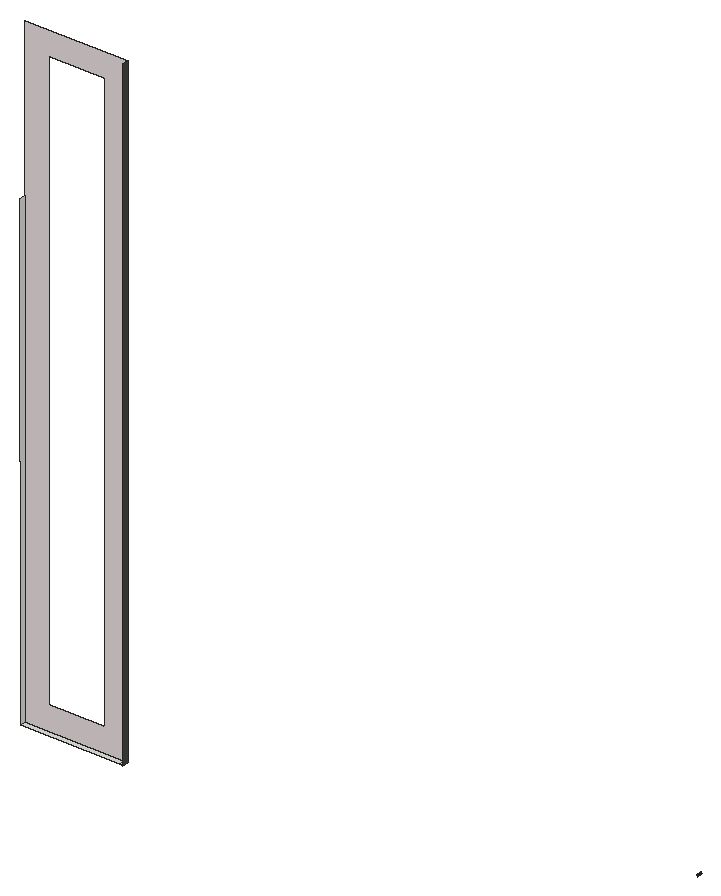
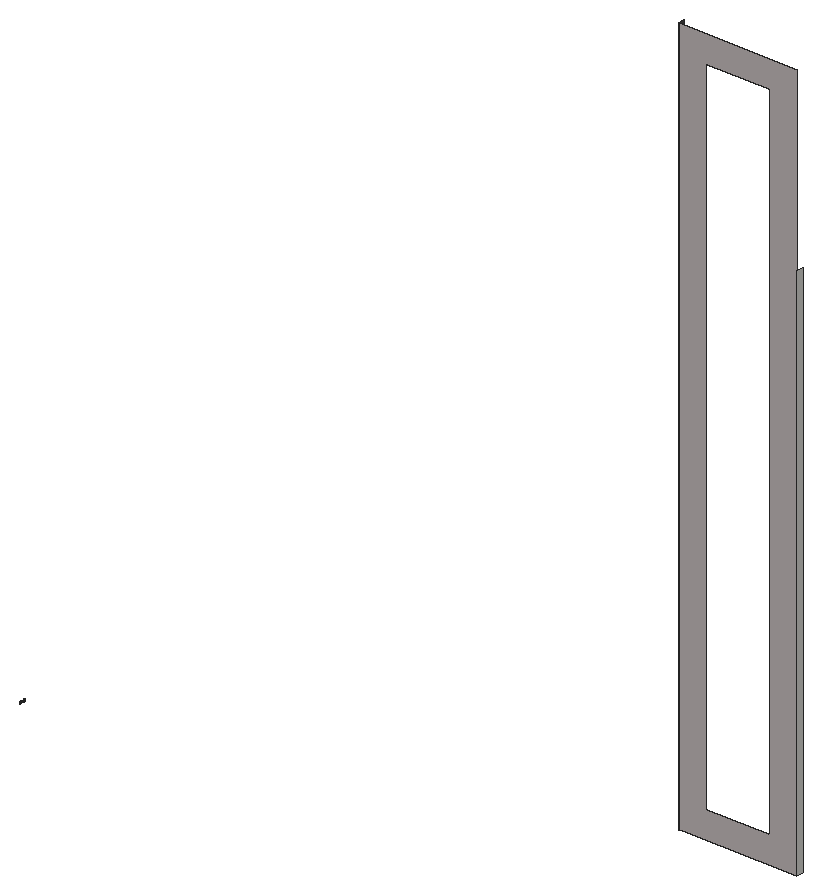
# SketchUp Ruby script. Lengths in inches.
U = 1.inch
M = Sketchup.active_model
def pt(a) = Geom::Point3d.new(a.map { |v| v * U })
def face(e, loops, mat)
  f = e.add_face(loops[0].map { |a| pt(a) })
  loops[1..].each { |l| e.add_face(l.map { |a| pt(a) }).erase! }
  f.material = f.back_material = mat if mat
  f
end
# faces: each face lists its corners as indices into pts; further lists are holes
def faces(e, pts, list, mat = nil) = list.each { |f| face(e, (f[0].is_a?(Array) ? f : [f]).map { |l| l.map { |i| pts[i] } }, mat) }
# xy, xz, yz: faces in a plane at the given z, y or x. An outline is a flat list of corners, or four numbers for a rectangle; further outlines are holes
def ring(l) = l.size == 4 ? [[l[0], l[1]], [l[2], l[1]], [l[2], l[3]], [l[0], l[3]]] : l.each_slice(2).to_a
def flat(e, list, mat, &to3) = list.each { |f| face(e, (f[0].is_a?(Array) ? f : [f]).map { |l| ring(l).map { |u, v| to3.(u, v) } }, mat) }
def xy(e, z, list, mat = nil) = flat(e, list, mat) { |x, y| [x, y, z] }
def xz(e, y, list, mat = nil) = flat(e, list, mat) { |x, z| [x, y, z] }
def yz(e, x, list, mat = nil) = flat(e, list, mat) { |y, z| [x, y, z] }
def lines(e, pts, list) = list.each { |a, b| e.add_line(pt(pts[a]), pt(pts[b])) }
# prism: a flat outline (further loops are holes) pulled along v
def prism(e, loops, v, mat = nil)
  f = face(e, loops, mat); d = Geom::Vector3d.new(v.map { |x| x * U })
  f.pushpull(f.normal.samedirection?(d) ? d.length : -d.length)
end
def box(e, o, s, mat = nil) = prism(e, [[o, [o[0] + s[0], o[1], o[2]], [o[0] + s[0], o[1] + s[1], o[2]], [o[0], o[1] + s[1], o[2]]]], [0, 0, s[2]], mat)
def at(x, y, z, deg = 0) = Geom::Transformation.translation(pt([x, y, z])) * Geom::Transformation.rotation(ORIGIN, Z_AXIS, deg.degrees)
def axes(o, x, y, z) = Geom::Transformation.new([*x, 0, *y, 0, *z, 0, *pt(o).to_a, 1])
def part(name) = M.definitions.add(name)
# library, detail: a bought-in or finely detailed component or shape, given as its bounding box
def library(name, o, s) = part(name).tap { |d| box(d.entities, o, s) }
def detail(e, o, s) = box(e.add_group.entities, o, s)
def put(e, d, t, mat = nil) = e.add_instance(d, t).tap { |i| i.material = mat if mat }
def group(e, t, mat = nil) = e.add_group.tap { |g| g.transformation = t; g.material = mat if mat }.entities
root = M.entities
M.materials.add("Generic\#1").color = [73, 71, 71]
M.materials.add("Generic\#5").color = [232, 222, 222]
M.materials.add("Material \#1").color = [140, 140, 140]
xy(root,30.535,[[34.973,39.25,88.165,42.5],[88.165,39.25,90.291,42.5]])
xy(root,30.853,[[337.189,118.4375,337.249,118.786,337.189,118.786]],"Material \#1")
xz(root,42.5,[[[34.973,30.535,90.291,30.535,90.279,368.38,34.912,368.38,34.917,283.879],[47.667,43.231,47.614,283.881,47.609,355.683,77.584,355.683,77.594,43.231]]],"Generic\#5")
xz(root,116.525,[[337.219,29.939,337.096,30,337.341,30],[337.219,29.939,337.15,29.955,337.096,30],[337.219,29.939,337.183,29.943,337.15,29.955],[337.15,29.955,337.121,29.974,337.096,30],[337.341,30,336.94,30.643,337.025,30.52],
  [337.341,30,337.056,30.439,336.94,30.643],[337.096,30,337.061,30.42,337.341,30],[337.096,30,337.062,30.414,337.061,30.42],[337.096,30,337.066,30.064,337.062,30.414],[337.096,30,337.078,30.03,337.066,30.064],
  [337.341,30,337.11,30.45,337.162,30.431],[337.066,30.064,337.062,30.102,337.062,30.414],[337.056,30.439,337.052,30.444,336.94,30.643],[337.052,30.444,337.048,30.45,336.94,30.643],[337.048,30.45,336.994,30.507,336.94,30.643],
  [337.048,30.45,337.043,30.455,336.994,30.507],[337.043,30.455,337.017,30.479,336.994,30.507],[336.994,30.507,336.959,30.57,336.94,30.643],[336.994,30.507,336.975,30.537,336.959,30.57],[337.025,30.52,336.94,30.643,336.996,30.568],
  [336.996,30.568,336.94,30.643,336.978,30.622],[336.959,30.57,336.948,30.606,336.94,30.643],[336.978,30.622,336.94,30.643,336.971,30.681],[336.94,30.643,336.938,30.681,336.945,30.748],[336.94,30.643,336.945,30.748,337,30.864],
  [336.94,30.643,336.978,30.74,336.971,30.681],[336.94,30.643,337,30.864,336.978,30.74],[336.978,30.74,337,30.864,336.996,30.795],[336.945,30.748,336.967,30.81,337,30.864],[336.996,30.795,337,30.864,337.025,30.842],
  [337.025,30.842,337,30.864,337.064,30.882],[337,30.864,337.043,30.909,337.095,30.944],[337,30.864,337.095,30.944,337.219,30.973],[337,30.864,337.11,30.913,337.064,30.882],[337,30.864,337.219,30.973,337.11,30.913],
  [337.11,30.913,337.219,30.973,337.162,30.932],[337.162,30.932,337.219,30.973,337.219,30.939],[337.095,30.944,337.154,30.966,337.219,30.973]],"Material \#1")
xz(root,116.862,[[337.207,30.51,337.195,30.535,337.231,30.535],[337.207,30.51,337.231,30.535,337.243,30.51],[337.195,30.535,337.189,30.544,337.237,30.544],[337.195,30.535,337.237,30.544,337.231,30.535],[337.189,30.544,337.189,30.563,337.237,30.563],
  [337.189,30.544,337.237,30.563,337.237,30.544],[337.189,30.563,337.195,30.572,337.231,30.572],[337.189,30.563,337.231,30.572,337.237,30.563],[337.195,30.572,337.195,30.604,337.243,30.604],[337.195,30.572,337.243,30.604,337.231,30.572],
  [337.195,30.604,337.195,30.634,337.243,30.634],[337.195,30.604,337.243,30.634,337.243,30.604],[337.195,30.634,337.186,30.658,337.252,30.658],[337.195,30.634,337.252,30.658,337.243,30.634],[337.186,30.658,337.186,30.683,337.252,30.683],
  [337.186,30.658,337.252,30.683,337.252,30.658],[337.186,30.683,337.195,30.707,337.243,30.707],[337.186,30.683,337.243,30.707,337.252,30.683],[337.195,30.707,337.189,30.724,337.249,30.724],[337.195,30.707,337.249,30.724,337.243,30.707],
  [337.189,30.724,337.189,30.78,337.249,30.78],[337.189,30.724,337.249,30.78,337.249,30.724],[337.189,30.78,337.196,30.784,337.241,30.784],[337.189,30.78,337.241,30.784,337.249,30.78],[337.196,30.784,337.196,30.793,337.241,30.793],
  [337.196,30.784,337.241,30.793,337.241,30.784],[337.196,30.793,337.189,30.797,337.249,30.797],[337.196,30.793,337.249,30.797,337.241,30.793],[337.189,30.797,337.189,30.853,337.249,30.853],[337.189,30.797,337.249,30.853,337.249,30.797]],"Material \#1")
xz(root,116.9,[[337.219,29.939,337.15,29.955,337.183,29.943],[337.15,29.955,337.062,30.414,337.066,30.064],[337.15,29.955,337.371,30.064,337.062,30.414],[337.15,29.955,337.066,30.064,337.096,30],[337.15,29.955,337.096,30,337.121,29.974],
  [337.096,30,337.066,30.064,337.078,30.03],[337.371,30.064,337.056,30.439,337.058,30.433],[337.371,30.064,337.058,30.433,337.06,30.427],[337.371,30.064,337.06,30.427,337.061,30.42],[337.371,30.064,337.061,30.42,337.062,30.414],
  [337.066,30.064,337.062,30.414,337.062,30.102],[337.375,30.102,337.025,30.52,337.056,30.439],[337.375,30.102,337.064,30.48,337.025,30.52],[337.375,30.102,337.11,30.45,337.064,30.48],[337.375,30.102,337.162,30.431,337.11,30.45],
  [337.056,30.439,336.94,30.643,337.052,30.444],[337.056,30.439,336.996,30.568,336.94,30.643],[337.056,30.439,337.025,30.52,336.996,30.568],[337.052,30.444,336.94,30.643,337.048,30.45],[337.048,30.45,336.94,30.643,336.994,30.507],
  [337.048,30.45,336.994,30.507,337.043,30.455],[337.043,30.455,336.994,30.507,337.017,30.479],[336.994,30.507,336.94,30.643,336.959,30.57],[336.994,30.507,336.959,30.57,336.975,30.537],[336.996,30.568,336.978,30.622,336.94,30.643],
  [336.959,30.57,336.94,30.643,336.948,30.606],[336.978,30.622,336.971,30.681,336.94,30.643],[336.94,30.643,336.945,30.748,336.938,30.681],[336.94,30.643,336.971,30.681,336.978,30.74],[336.94,30.643,336.978,30.74,336.996,30.795],
  [336.94,30.643,336.996,30.795,337,30.864],[336.94,30.643,337,30.864,336.945,30.748],[336.945,30.748,337,30.864,336.967,30.81],[336.996,30.795,337.025,30.842,337,30.864],[337.025,30.842,337.064,30.882,337,30.864],
  [337,30.864,337.064,30.882,337.11,30.913],[337,30.864,337.095,30.944,337.043,30.909],[337,30.864,337.11,30.913,337.219,30.973],[337,30.864,337.219,30.973,337.095,30.944],[337.11,30.913,337.162,30.932,337.219,30.973],
  [337.162,30.932,337.219,30.939,337.219,30.973],[337.095,30.944,337.219,30.973,337.154,30.966]],"Material \#1")
xz(root,118.4,[[337.219,29.939,337.15,29.955,337.288,29.955],[337.219,29.939,337.183,29.943,337.15,29.955],[337.15,29.955,337.062,30.414,337.371,30.064],[337.15,29.955,337.066,30.064,337.062,30.414],[337.15,29.955,337.096,30,337.066,30.064],
  [337.15,29.955,337.121,29.974,337.096,30],[337.096,30,337.078,30.03,337.066,30.064],[337.371,30.064,337.058,30.433,337.056,30.439],[337.371,30.064,337.06,30.427,337.058,30.433],[337.371,30.064,337.061,30.42,337.06,30.427],
  [337.371,30.064,337.062,30.414,337.061,30.42],[337.066,30.064,337.062,30.102,337.062,30.414],[337.375,30.102,337.025,30.52,337.064,30.48],[337.375,30.102,337.056,30.439,337.025,30.52],[337.375,30.102,337.064,30.48,337.11,30.45],
  [337.375,30.102,337.11,30.45,337.162,30.431],[337.056,30.439,336.94,30.643,336.996,30.568],[337.056,30.439,337.052,30.444,336.94,30.643],[337.056,30.439,336.996,30.568,337.025,30.52],[337.052,30.444,337.048,30.45,336.94,30.643],
  [337.048,30.45,336.994,30.507,336.94,30.643],[337.048,30.45,337.043,30.455,336.994,30.507],[337.043,30.455,337.017,30.479,336.994,30.507],[336.994,30.507,336.959,30.57,336.94,30.643],[336.994,30.507,336.975,30.537,336.959,30.57],
  [336.996,30.568,336.94,30.643,336.978,30.622],[336.959,30.57,336.948,30.606,336.94,30.643],[336.978,30.622,336.94,30.643,336.971,30.681],[336.94,30.643,336.938,30.681,336.945,30.748],[336.94,30.643,336.945,30.748,337,30.864],
  [336.94,30.643,336.978,30.74,336.971,30.681],[336.94,30.643,336.996,30.795,336.978,30.74],[336.94,30.643,337,30.864,336.996,30.795],[336.945,30.748,336.967,30.81,337,30.864],[336.996,30.795,337,30.864,337.025,30.842],
  [337.025,30.842,337,30.864,337.064,30.882],[337,30.864,337.043,30.909,337.095,30.944],[337,30.864,337.095,30.944,337.219,30.973],[337,30.864,337.11,30.913,337.064,30.882],[337,30.864,337.219,30.973,337.11,30.913],
  [337.11,30.913,337.219,30.973,337.162,30.932],[337.162,30.932,337.219,30.973,337.219,30.939],[337.095,30.944,337.154,30.966,337.219,30.973]],"Material \#1")
xz(root,118.4375,[[337.207,30.51,337.231,30.535,337.195,30.535],[337.207,30.51,337.243,30.51,337.231,30.535],[337.195,30.535,337.237,30.544,337.189,30.544],[337.195,30.535,337.231,30.535,337.237,30.544],[337.189,30.544,337.237,30.544,337.237,30.563],
  [337.189,30.544,337.237,30.563,337.189,30.563],[337.189,30.563,337.231,30.572,337.195,30.572],[337.189,30.563,337.237,30.563,337.231,30.572],[337.195,30.572,337.231,30.572,337.243,30.604],[337.195,30.572,337.243,30.604,337.195,30.604],
  [337.195,30.604,337.243,30.604,337.243,30.634],[337.195,30.604,337.243,30.634,337.195,30.634],[337.195,30.634,337.252,30.658,337.186,30.658],[337.195,30.634,337.243,30.634,337.252,30.658],[337.186,30.658,337.252,30.658,337.252,30.683],
  [337.186,30.658,337.252,30.683,337.186,30.683],[337.186,30.683,337.243,30.707,337.195,30.707],[337.186,30.683,337.252,30.683,337.243,30.707],[337.195,30.707,337.249,30.724,337.189,30.724],[337.195,30.707,337.243,30.707,337.249,30.724],
  [337.189,30.724,337.249,30.724,337.249,30.78],[337.189,30.724,337.249,30.78,337.189,30.78],[337.189,30.78,337.241,30.784,337.196,30.784],[337.189,30.78,337.249,30.78,337.241,30.784],[337.196,30.784,337.241,30.784,337.241,30.793],
  [337.196,30.784,337.241,30.793,337.196,30.793],[337.196,30.793,337.249,30.797,337.189,30.797],[337.196,30.793,337.241,30.793,337.249,30.797],[337.189,30.797,337.249,30.797,337.249,30.853],[337.189,30.797,337.249,30.853,337.189,30.853]],"Material \#1")
xz(root,118.775,[[337.219,29.939,337.096,30,337.15,29.955],[337.219,29.939,337.341,30,337.096,30],[337.219,29.939,337.15,29.955,337.183,29.943],[337.15,29.955,337.096,30,337.121,29.974],[337.341,30,336.94,30.643,337.056,30.439],
  [337.341,30,337.025,30.52,336.94,30.643],[337.341,30,337.064,30.48,337.025,30.52],[337.341,30,337.056,30.439,337.058,30.433],[337.341,30,337.058,30.433,337.06,30.427],[337.341,30,337.06,30.427,337.061,30.42],
  [337.096,30,337.061,30.42,337.062,30.414],[337.096,30,337.341,30,337.061,30.42],[337.096,30,337.062,30.414,337.066,30.064],[337.341,30,337.11,30.45,337.064,30.48],[337.096,30,337.066,30.064,337.078,30.03],
  [337.341,30,337.162,30.431,337.11,30.45],[337.066,30.064,337.062,30.414,337.062,30.102],[337.056,30.439,336.94,30.643,337.052,30.444],[337.052,30.444,336.94,30.643,337.048,30.45],[337.048,30.45,336.94,30.643,336.994,30.507],
  [337.048,30.45,336.994,30.507,337.043,30.455],[337.043,30.455,336.994,30.507,337.017,30.479],[336.994,30.507,336.94,30.643,336.959,30.57],[336.994,30.507,336.959,30.57,336.975,30.537],[337.025,30.52,336.996,30.568,336.94,30.643],
  [336.996,30.568,336.978,30.622,336.94,30.643],[336.959,30.57,336.94,30.643,336.948,30.606],[336.978,30.622,336.971,30.681,336.94,30.643],[336.94,30.643,336.945,30.748,336.938,30.681],[336.94,30.643,336.971,30.681,336.978,30.74],
  [336.94,30.643,336.978,30.74,337,30.864],[336.94,30.643,337,30.864,336.945,30.748],[336.978,30.74,336.996,30.795,337,30.864],[336.945,30.748,337,30.864,336.967,30.81],[336.996,30.795,337.025,30.842,337,30.864],
  [337.025,30.842,337.064,30.882,337,30.864],[337,30.864,337.064,30.882,337.11,30.913],[337,30.864,337.095,30.944,337.043,30.909],[337,30.864,337.11,30.913,337.219,30.973],[337,30.864,337.219,30.973,337.095,30.944],
  [337.11,30.913,337.162,30.932,337.219,30.973],[337.162,30.932,337.219,30.939,337.219,30.973],[337.095,30.944,337.219,30.973,337.154,30.966]],"Material \#1")
yz(root,337.189,[[116.862,30.797,116.513,30.853,116.862,30.853],[118.4375,30.797,118.4375,30.853,118.786,30.853]],"Material \#1")
yz(root,337.195,[[116.862,30.572,116.513,30.604,116.862,30.604],[118.4375,30.572,118.4375,30.604,118.786,30.604]],"Material \#1")
p = [[34.973,42.5,30.535],[34.917,42.5,283.879],[34.917,39.25,283.879],[34.973,39.25,30.535],[90.279,42.5,368.38],[90.291,42.5,30.535],
  [90.291,39.25,30.535],[90.279,39.25,368.38],[337.192,116.513,30.568],[337.189,116.862,30.563],[337.189,116.862,30.544],[337.192,116.513,30.54],
  [337.192,116.513,30.54],[337.189,116.862,30.544],[337.195,116.862,30.535],[337.192,116.513,30.54],[337.195,116.862,30.535],[337.207,116.862,30.51],
  [337.207,116.513,30.51],[337.192,116.513,30.54],[337.192,118.786,30.568],[337.192,118.786,30.54],[337.189,118.4375,30.544],[337.189,118.4375,30.563],
  [337.192,118.786,30.54],[337.195,118.4375,30.535],[337.189,118.4375,30.544],[337.192,118.786,30.54],[337.207,118.786,30.51],[337.207,118.4375,30.51],
  [337.195,118.4375,30.535],[337.192,118.786,30.54],[337.186,116.513,30.671],[337.186,116.862,30.658],[337.195,116.862,30.634],[337.195,116.862,30.634],
  [337.19,116.513,30.646],[337.186,116.513,30.671],[337.192,116.513,30.568],[337.195,116.862,30.572],[337.189,116.862,30.563],[337.19,116.513,30.646],
  [337.195,116.862,30.634],[337.195,116.862,30.604],[337.195,116.862,30.604],[337.195,116.513,30.604],[337.19,116.513,30.646],[337.195,116.862,30.572],
  [337.192,116.513,30.568],[337.195,116.513,30.604],[337.195,118.4375,30.634],[337.186,118.4375,30.658],[337.186,118.786,30.671],[337.186,118.786,30.671],
  [337.19,118.786,30.646],[337.195,118.4375,30.634],[337.192,118.786,30.568],[337.189,118.4375,30.563],[337.195,118.4375,30.572],[337.19,118.786,30.646],
  [337.195,118.786,30.604],[337.195,118.4375,30.604],[337.195,118.4375,30.604],[337.195,118.4375,30.634],[337.19,118.786,30.646],[337.195,118.786,30.604],
  [337.192,118.786,30.568],[337.195,118.4375,30.572],[337.19,116.513,30.695],[337.186,116.862,30.683],[337.186,116.862,30.658],[337.186,116.862,30.658],
  [337.186,116.513,30.671],[337.19,116.513,30.695],[337.186,116.862,30.683],[337.19,116.513,30.695],[337.192,116.513,30.716],[337.192,116.513,30.785],
  [337.189,116.862,30.78],[337.189,116.862,30.724],[337.189,116.862,30.724],[337.189,116.513,30.728],[337.192,116.513,30.785],[337.192,116.513,30.716],
  [337.195,116.862,30.707],[337.186,116.862,30.683],[337.189,116.513,30.728],[337.189,116.862,30.724],[337.195,116.862,30.707],[337.195,116.862,30.707],
  [337.192,116.513,30.716],[337.189,116.513,30.728],[337.186,118.4375,30.658],[337.186,118.4375,30.683],[337.19,118.786,30.695],[337.19,118.786,30.695],
  [337.186,118.786,30.671],[337.186,118.4375,30.658],[337.192,118.786,30.716],[337.19,118.786,30.695],[337.186,118.4375,30.683],[337.189,118.4375,30.724],
  [337.189,118.4375,30.78],[337.192,118.786,30.785],[337.192,118.786,30.785],[337.189,118.786,30.728],[337.189,118.4375,30.724],[337.186,118.4375,30.683],
  [337.195,118.4375,30.707],[337.192,118.786,30.716],[337.195,118.4375,30.707],[337.189,118.4375,30.724],[337.189,118.786,30.728],[337.189,118.786,30.728],
  [337.192,118.786,30.716],[337.195,118.4375,30.707],[337.189,116.862,30.797],[337.192,116.513,30.785],[337.189,116.513,30.853],[337.246,116.513,30.791],
  [337.249,116.862,30.78],[337.241,116.862,30.784],[337.192,116.513,30.785],[337.196,116.862,30.793],[337.196,116.862,30.784],[337.192,116.513,30.785],
  [337.189,116.862,30.797],[337.192,116.513,30.785],[337.189,116.862,30.78],[337.246,116.513,30.791],[337.241,116.862,30.793],[337.249,116.862,30.797],
  [337.246,116.513,30.791],[337.189,118.786,30.853],[337.192,118.786,30.785],[337.189,118.4375,30.797],[337.246,118.786,30.791],[337.241,118.4375,30.784],
  [337.249,118.4375,30.78],[337.192,118.786,30.785],[337.196,118.4375,30.784],[337.196,118.4375,30.793],[337.192,118.786,30.785],[337.189,118.4375,30.797],
  [337.192,118.786,30.785],[337.189,118.4375,30.78],[337.246,118.786,30.791],[337.249,118.4375,30.797],[337.241,118.4375,30.793],[337.246,118.786,30.791]]
faces(root,p,[[0,1,2,3]])
faces(root,p,[[4,5,6,7]],"Generic\#1")
faces(root,p,[[8,9,10],[10,11,8],[12,13,14],[15,16,17],[17,18,19],[20,21,22],[22,23,20],[24,25,26],
  [27,28,29],[29,30,31],[32,33,34],[35,36,37],[38,39,40],[41,42,43],[44,45,46],[47,48,49],
  [50,51,52],[53,54,55],[56,57,58],[59,60,61],[62,63,64],[65,66,67],[68,69,70],[71,72,73],
  [74,75,76],[77,78,79],[80,81,82],[83,84,85],[86,87,88],[89,90,91],[92,93,94],[95,96,97],
  [98,99,100],[101,102,103],[104,105,106],[107,108,109],[110,111,112],[113,114,115],[116,117,118],[119,120,121],
  [122,123,124],[125,126,123],[127,124,128],[129,130,131],[132,121,130],[133,134,135],[136,137,138],[139,140,141],
  [142,141,143],[144,145,140],[146,147,148],[149,148,137]],"Material \#1")
